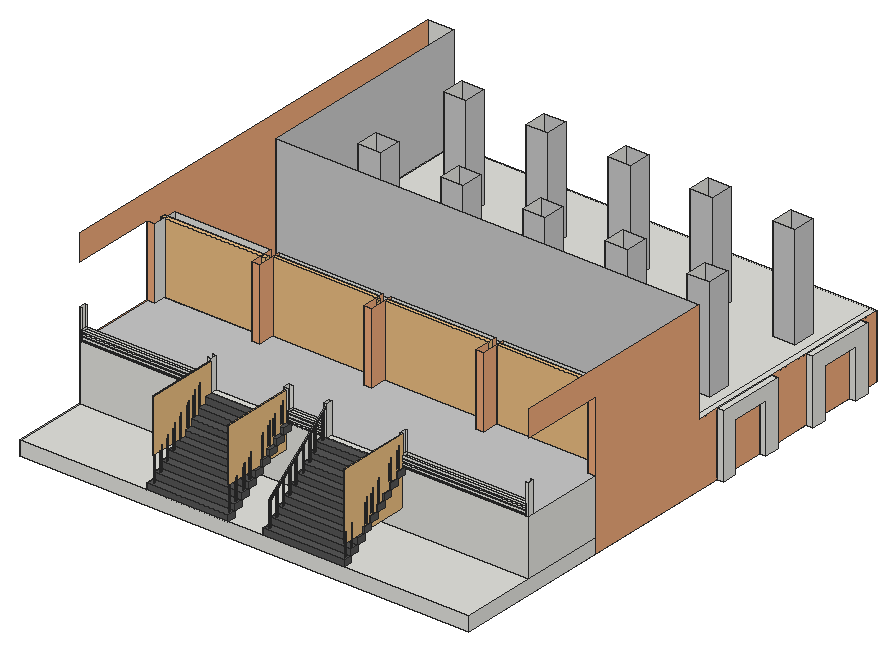
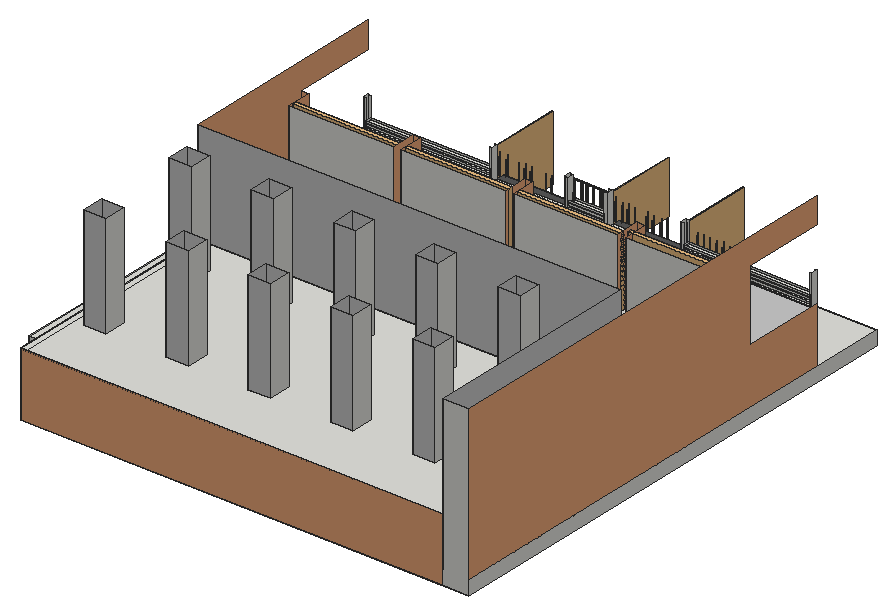
# SketchUp Ruby script. Lengths in inches.
U = 1.inch
M = Sketchup.active_model
def pt(a) = Geom::Point3d.new(a.map { |v| v * U })
def face(e, loops, mat)
  f = e.add_face(loops[0].map { |a| pt(a) })
  loops[1..].each { |l| e.add_face(l.map { |a| pt(a) }).erase! }
  f.material = f.back_material = mat if mat
  f
end
# faces: each face lists its corners as indices into pts; further lists are holes
def faces(e, pts, list, mat = nil) = list.each { |f| face(e, (f[0].is_a?(Array) ? f : [f]).map { |l| l.map { |i| pts[i] } }, mat) }
# xy, xz, yz: faces in a plane at the given z, y or x. An outline is a flat list of corners, or four numbers for a rectangle; further outlines are holes
def ring(l) = l.size == 4 ? [[l[0], l[1]], [l[2], l[1]], [l[2], l[3]], [l[0], l[3]]] : l.each_slice(2).to_a
def flat(e, list, mat, &to3) = list.each { |f| face(e, (f[0].is_a?(Array) ? f : [f]).map { |l| ring(l).map { |u, v| to3.(u, v) } }, mat) }
def xy(e, z, list, mat = nil) = flat(e, list, mat) { |x, y| [x, y, z] }
def xz(e, y, list, mat = nil) = flat(e, list, mat) { |x, z| [x, y, z] }
def yz(e, x, list, mat = nil) = flat(e, list, mat) { |y, z| [x, y, z] }
def lines(e, pts, list) = list.each { |a, b| e.add_line(pt(pts[a]), pt(pts[b])) }
# prism: a flat outline (further loops are holes) pulled along v
def prism(e, loops, v, mat = nil)
  f = face(e, loops, mat); d = Geom::Vector3d.new(v.map { |x| x * U })
  f.pushpull(f.normal.samedirection?(d) ? d.length : -d.length)
end
def box(e, o, s, mat = nil) = prism(e, [[o, [o[0] + s[0], o[1], o[2]], [o[0] + s[0], o[1] + s[1], o[2]], [o[0], o[1] + s[1], o[2]]]], [0, 0, s[2]], mat)
def at(x, y, z, deg = 0) = Geom::Transformation.translation(pt([x, y, z])) * Geom::Transformation.rotation(ORIGIN, Z_AXIS, deg.degrees)
def axes(o, x, y, z) = Geom::Transformation.new([*x, 0, *y, 0, *z, 0, *pt(o).to_a, 1])
def part(name) = M.definitions.add(name)
# library, detail: a bought-in or finely detailed component or shape, given as its bounding box
def library(name, o, s) = part(name).tap { |d| box(d.entities, o, s) }
def detail(e, o, s) = box(e.add_group.entities, o, s)
def put(e, d, t, mat = nil) = e.add_instance(d, t).tap { |i| i.material = mat if mat }
def group(e, t, mat = nil) = e.add_group.tap { |g| g.transformation = t; g.material = mat if mat }.entities
root = M.entities
M.materials.add("Generic\#1").color = [236, 168, 122]
M.materials.add("Generic\#4").color = [201, 201, 201]
M.materials.add("[Color M06]").color = [86, 86, 86]
c1 = part("Group\#6")
xy(c1.entities,0,[[0,0,123.875,12.625]])
xy(c1.entities,9.4375,[[0,0,123.875,12.625]])
xz(c1.entities,0,[[0,0,123.875,9.4375]])
yz(c1.entities,0,[[0,0,12.625,9.4375]])
yz(c1.entities,123.875,[[0,0,12.625,9.4375]])
c2 = library("Group\#7",[0,0,0],[158.4375,6,107.5625])
prism(root,[[[214.39,5.8,-54.75],[214.29,6.05,-54.75],[214.26,6.3,-54.75],[214.29,6.5625,-54.75],[214.39,6.8,-54.75],[214.55,7.01,-54.75],[214.76,7.17,-54.75],[215,7.27,-54.75],[215.26,7.3,-54.75],[215.52,7.27,-54.75],[215.76,7.17,-54.75],[215.97,7.01,-54.75],[216.125,6.8,-54.75],[216.23,6.5625,-54.75],[216.26,6.3,-54.75],[216.23,6.05,-54.75],[216.125,5.8,-54.75],[215.97,5.6,-54.75],[215.76,5.4375,-54.75],[215.52,5.34,-54.75],[215.26,5.3,-54.75],[215,5.34,-54.75],[214.76,5.4375,-54.75],[214.55,5.6,-54.75]]],[0,0,37.69])
prism(root,[[[329.63,5.9375,-54.75],[329.39,5.84,-54.75],[329.13,5.8,-54.75],[328.875,5.84,-54.75],[328.63,5.9375,-54.75],[328.43,6.1,-54.75],[328.27,6.3,-54.75],[328.17,6.55,-54.75],[328.13,6.8,-54.75],[328.17,7.0625,-54.75],[328.27,7.3,-54.75],[328.43,7.51,-54.75],[328.63,7.67,-54.75],[328.875,7.77,-54.75],[329.13,7.8,-54.75],[329.39,7.77,-54.75],[329.63,7.67,-54.75],[329.84,7.51,-54.75],[330,7.3,-54.75],[330.1,7.0625,-54.75],[330.13,6.8,-54.75],[330.1,6.55,-54.75],[330,6.3,-54.75],[329.84,6.1,-54.75]]],[0,0,38.25])
prism(root,[[[390.83,7.14,-54.75],[391.07,7.25,-54.75],[391.32,7.3,-54.75],[391.58,7.28,-54.75],[391.83,7.2,-54.75],[392.05,7.05,-54.75],[392.22,6.86,-54.75],[392.33,6.625,-54.75],[392.38,6.37,-54.75],[392.36,6.11,-54.75],[392.28,5.86,-54.75],[392.13,5.64,-54.75],[391.9375,5.47,-54.75],[391.7,5.36,-54.75],[391.45,5.31,-54.75],[391.1875,5.32,-54.75],[390.94,5.41,-54.75],[390.72,5.55,-54.75],[390.55,5.75,-54.75],[390.4375,5.98,-54.75],[390.39,6.24,-54.75],[390.4,6.5,-54.75],[390.49,6.75,-54.75],[390.63,6.97,-54.75]]],[0,0,38.17])
prism(root,[[[505.97,6.1,-54.75],[505.76,5.9375,-54.75],[505.52,5.84,-54.75],[505.26,5.8,-54.75],[505,5.84,-54.75],[504.76,5.9375,-54.75],[504.55,6.1,-54.75],[504.39,6.3,-54.75],[504.29,6.55,-54.75],[504.26,6.8,-54.75],[504.29,7.0625,-54.75],[504.39,7.3,-54.75],[504.55,7.51,-54.75],[504.76,7.67,-54.75],[505,7.77,-54.75],[505.26,7.8,-54.75],[505.52,7.77,-54.75],[505.76,7.67,-54.75],[505.97,7.51,-54.75],[506.125,7.3,-54.75],[506.23,7.0625,-54.75],[506.26,6.8,-54.75],[506.23,6.55,-54.75],[506.125,6.3,-54.75]]],[0,0,38.28])
prism(root,[[[214.55,18.28,-45.3125],[214.39,18.49,-45.3125],[214.29,18.73,-45.3125],[214.26,18.99,-45.3125],[214.29,19.25,-45.3125],[214.39,19.49,-45.3125],[214.55,19.7,-45.3125],[214.76,19.86,-45.3125],[215,19.96,-45.3125],[215.26,19.99,-45.3125],[215.52,19.96,-45.3125],[215.76,19.86,-45.3125],[215.97,19.7,-45.3125],[216.125,19.49,-45.3125],[216.22,19.25,-45.3125],[216.26,18.99,-45.3125],[216.22,18.73,-45.3125],[216.125,18.49,-45.3125],[215.97,18.28,-45.3125],[215.76,18.125,-45.3125],[215.52,18.03,-45.3125],[215.26,17.99,-45.3125],[215,18.03,-45.3125],[214.76,18.125,-45.3125]]],[0,0,36.6875])
prism(root,[[[329.39,17.59,-45.3125],[329.13,17.55,-45.3125],[328.875,17.59,-45.3125],[328.63,17.6875,-45.3125],[328.43,17.85,-45.3125],[328.27,18.05,-45.3125],[328.17,18.3,-45.3125],[328.13,18.55,-45.3125],[328.17,18.8125,-45.3125],[328.27,19.05,-45.3125],[328.43,19.26,-45.3125],[328.63,19.42,-45.3125],[328.875,19.52,-45.3125],[329.13,19.55,-45.3125],[329.39,19.52,-45.3125],[329.63,19.42,-45.3125],[329.84,19.26,-45.3125],[330,19.05,-45.3125],[330.1,18.8125,-45.3125],[330.13,18.55,-45.3125],[330.1,18.3,-45.3125],[330,18.05,-45.3125],[329.84,17.85,-45.3125],[329.63,17.6875,-45.3125]]],[0,0,36.6875])
prism(root,[[[390.68,19.7,-45.3125],[390.88,19.86,-45.3125],[391.125,19.96,-45.3125],[391.38,19.99,-45.3125],[391.64,19.96,-45.3125],[391.88,19.86,-45.3125],[392.09,19.7,-45.3125],[392.25,19.49,-45.3125],[392.35,19.25,-45.3125],[392.38,18.99,-45.3125],[392.35,18.73,-45.3125],[392.25,18.49,-45.3125],[392.09,18.28,-45.3125],[391.88,18.125,-45.3125],[391.64,18.03,-45.3125],[391.38,17.99,-45.3125],[391.125,18.03,-45.3125],[390.88,18.125,-45.3125],[390.68,18.28,-45.3125],[390.52,18.49,-45.3125],[390.42,18.73,-45.3125],[390.38,18.99,-45.3125],[390.42,19.25,-45.3125],[390.52,19.49,-45.3125]]],[0,0,37.04])
prism(root,[[[505.26,17.55,-45.3125],[505,17.59,-45.3125],[504.76,17.6875,-45.3125],[504.55,17.85,-45.3125],[504.39,18.05,-45.3125],[504.29,18.3,-45.3125],[504.26,18.55,-45.3125],[504.29,18.8125,-45.3125],[504.39,19.05,-45.3125],[504.55,19.26,-45.3125],[504.76,19.42,-45.3125],[505,19.52,-45.3125],[505.26,19.55,-45.3125],[505.52,19.52,-45.3125],[505.76,19.42,-45.3125],[505.97,19.26,-45.3125],[506.125,19.05,-45.3125],[506.22,18.8125,-45.3125],[506.26,18.55,-45.3125],[506.22,18.3,-45.3125],[506.125,18.05,-45.3125],[505.97,17.85,-45.3125],[505.76,17.6875,-45.3125],[505.52,17.59,-45.3125]]],[0,0,36.61])
prism(root,[[[216.26,31.24,-35.875],[216.22,30.98,-35.875],[216.125,30.74,-35.875],[215.96,30.53,-35.875],[215.76,30.375,-35.875],[215.52,30.28,-35.875],[215.26,30.24,-35.875],[215,30.28,-35.875],[214.76,30.375,-35.875],[214.55,30.53,-35.875],[214.39,30.74,-35.875],[214.29,30.98,-35.875],[214.26,31.24,-35.875],[214.29,31.5,-35.875],[214.39,31.74,-35.875],[214.55,31.95,-35.875],[214.76,32.11,-35.875],[215,32.21,-35.875],[215.26,32.24,-35.875],[215.52,32.21,-35.875],[215.76,32.11,-35.875],[215.96,31.95,-35.875],[216.125,31.74,-35.875],[216.22,31.5,-35.875]]],[0,0,36.6875])
prism(root,[[[329.39,34.64,-35.875],[329.63,34.54,-35.875],[329.84,34.39,-35.875],[330,34.18,-35.875],[330.1,33.9375,-35.875],[330.13,33.68,-35.875],[330.1,33.42,-35.875],[330,33.18,-35.875],[329.84,32.97,-35.875],[329.63,32.8125,-35.875],[329.39,32.71,-35.875],[329.13,32.68,-35.875],[328.875,32.71,-35.875],[328.63,32.8125,-35.875],[328.43,32.97,-35.875],[328.27,33.18,-35.875],[328.17,33.42,-35.875],[328.13,33.68,-35.875],[328.17,33.9375,-35.875],[328.27,34.18,-35.875],[328.43,34.39,-35.875],[328.63,34.54,-35.875],[328.875,34.64,-35.875],[329.13,34.68,-35.875]]],[0,0,38.36])
prism(root,[[[392.11,31.93,-35.875],[392.26,31.72,-35.875],[392.35,31.47,-35.875],[392.38,31.22,-35.875],[392.34,30.96,-35.875],[392.24,30.72,-35.875],[392.07,30.52,-35.875],[391.86,30.36,-35.875],[391.62,30.27,-35.875],[391.36,30.24,-35.875],[391.1,30.28,-35.875],[390.86,30.39,-35.875],[390.66,30.55,-35.875],[390.5,30.76,-35.875],[390.41,31.01,-35.875],[390.38,31.27,-35.875],[390.42,31.52,-35.875],[390.53,31.76,-35.875],[390.69,31.97,-35.875],[390.91,32.12,-35.875],[391.15,32.21,-35.875],[391.41,32.24,-35.875],[391.67,32.2,-35.875],[391.9,32.09,-35.875]]],[0,0,36.39])
prism(root,[[[215,43.02,-26.4375],[214.76,43.125,-26.4375],[214.55,43.28,-26.4375],[214.39,43.49,-26.4375],[214.29,43.73,-26.4375],[214.26,43.99,-26.4375],[214.29,44.25,-26.4375],[214.39,44.49,-26.4375],[214.55,44.7,-26.4375],[214.76,44.86,-26.4375],[215,44.96,-26.4375],[215.26,44.99,-26.4375],[215.52,44.96,-26.4375],[215.76,44.86,-26.4375],[215.96,44.7,-26.4375],[216.12,44.49,-26.4375],[216.22,44.25,-26.4375],[216.26,43.99,-26.4375],[216.22,43.73,-26.4375],[216.12,43.49,-26.4375],[215.96,43.28,-26.4375],[215.76,43.125,-26.4375],[215.52,43.02,-26.4375],[215.26,42.99,-26.4375]]],[0,0,36.6875])
prism(root,[[[328.13,45.68,-26.4375],[328.17,45.9375,-26.4375],[328.27,46.18,-26.4375],[328.42,46.39,-26.4375],[328.63,46.54,-26.4375],[328.87,46.64,-26.4375],[329.13,46.68,-26.4375],[329.39,46.64,-26.4375],[329.63,46.54,-26.4375],[329.84,46.39,-26.4375],[330,46.18,-26.4375],[330.1,45.9375,-26.4375],[330.13,45.68,-26.4375],[330.1,45.42,-26.4375],[330,45.18,-26.4375],[329.84,44.97,-26.4375],[329.63,44.8125,-26.4375],[329.39,44.71,-26.4375],[329.13,44.68,-26.4375],[328.87,44.71,-26.4375],[328.63,44.8125,-26.4375],[328.42,44.97,-26.4375],[328.27,45.18,-26.4375],[328.17,45.42,-26.4375]]],[0,0,38.36])
prism(root,[[[391.38,42.99,-26.4375],[391.12,43.02,-26.4375],[390.88,43.125,-26.4375],[390.67,43.28,-26.4375],[390.52,43.49,-26.4375],[390.42,43.73,-26.4375],[390.38,43.99,-26.4375],[390.42,44.25,-26.4375],[390.52,44.49,-26.4375],[390.67,44.7,-26.4375],[390.88,44.86,-26.4375],[391.12,44.96,-26.4375],[391.38,44.99,-26.4375],[391.64,44.96,-26.4375],[391.88,44.86,-26.4375],[392.09,44.7,-26.4375],[392.25,44.49,-26.4375],[392.35,44.25,-26.4375],[392.38,43.99,-26.4375],[392.35,43.73,-26.4375],[392.25,43.49,-26.4375],[392.09,43.28,-26.4375],[391.88,43.125,-26.4375],[391.64,43.02,-26.4375]]],[0,0,37.3125])
prism(root,[[[506.22,45.9375,-26.4375],[506.26,45.68,-26.4375],[506.22,45.42,-26.4375],[506.12,45.18,-26.4375],[505.96,44.97,-26.4375],[505.76,44.8125,-26.4375],[505.52,44.71,-26.4375],[505.26,44.68,-26.4375],[505,44.71,-26.4375],[504.76,44.8125,-26.4375],[504.55,44.97,-26.4375],[504.39,45.18,-26.4375],[504.29,45.42,-26.4375],[504.26,45.68,-26.4375],[504.29,45.9375,-26.4375],[504.39,46.18,-26.4375],[504.55,46.39,-26.4375],[504.76,46.54,-26.4375],[505,46.64,-26.4375],[505.26,46.68,-26.4375],[505.52,46.64,-26.4375],[505.76,46.54,-26.4375],[505.96,46.39,-26.4375],[506.12,46.18,-26.4375]]],[0,0,37.92])
prism(root,[[[391.77,6.06,-17.3],[391.96,6,-17.22],[392.11,5.93,-17.13],[392.19,5.85,-17.02],[392.22,5.76,-16.9],[392.18,5.68,-16.78],[392.08,5.6,-16.67],[391.92,5.53,-16.58],[391.72,5.47,-16.51],[391.49,5.44,-16.47],[391.24,5.43,-16.46],[391,5.44,-16.48],[390.77,5.48,-16.52],[390.58,5.53,-16.6],[390.43,5.6,-16.7],[390.34,5.6875,-16.81],[390.32,5.77,-16.92],[390.35,5.86,-17.04],[390.46,5.94,-17.15],[390.61,6.01,-17.24],[390.8125,6.0625,-17.3125],[391.05,6.09,-17.35],[391.29,6.1,-17.37],[391.54,6.09,-17.35]]],[-0.53,106.82,78.87])
prism(root,[[[215.96,55.03,-17],[215.76,54.875,-17],[215.51,54.77,-17],[215.26,54.74,-17],[215,54.77,-17],[214.76,54.875,-17],[214.55,55.03,-17],[214.39,55.24,-17],[214.29,55.48,-17],[214.26,55.74,-17],[214.29,56,-17],[214.39,56.24,-17],[214.55,56.45,-17],[214.76,56.61,-17],[215,56.71,-17],[215.26,56.74,-17],[215.51,56.71,-17],[215.76,56.61,-17],[215.96,56.45,-17],[216.12,56.24,-17],[216.22,56,-17],[216.26,55.74,-17],[216.22,55.48,-17],[216.12,55.24,-17]]],[0,0,36.25])
prism(root,[[[504.76,56.8125,-17],[504.55,56.97,-17],[504.39,57.18,-17],[504.29,57.42,-17],[504.26,57.68,-17],[504.29,57.9375,-17],[504.39,58.18,-17],[504.55,58.39,-17],[504.76,58.54,-17],[505,58.64,-17],[505.26,58.68,-17],[505.51,58.64,-17],[505.76,58.54,-17],[505.96,58.39,-17],[506.12,58.18,-17],[506.22,57.9375,-17],[506.26,57.68,-17],[506.22,57.42,-17],[506.12,57.18,-17],[505.96,56.97,-17],[505.76,56.8125,-17],[505.51,56.71,-17],[505.26,56.68,-17],[505,56.71,-17]]],[0,0,37.02])
prism(root,[[[392.25,55.24,-17],[392.09,55.03,-17],[391.88,54.875,-17],[391.64,54.77,-17],[391.38,54.74,-17],[391.12,54.77,-17],[390.88,54.875,-17],[390.67,55.03,-17],[390.51,55.24,-17],[390.41,55.48,-17],[390.38,55.74,-17],[390.41,56,-17],[390.51,56.24,-17],[390.67,56.45,-17],[390.88,56.61,-17],[391.12,56.71,-17],[391.38,56.74,-17],[391.64,56.71,-17],[391.88,56.61,-17],[392.09,56.45,-17],[392.25,56.24,-17],[392.35,56,-17],[392.38,55.74,-17],[392.35,55.48,-17]]],[0,0,35.9375])
prism(root,[[[215,68.71,-7.5625],[214.75,68.8125,-7.5625],[214.55,68.97,-7.5625],[214.39,69.18,-7.5625],[214.29,69.42,-7.5625],[214.25,69.68,-7.5625],[214.29,69.9375,-7.5625],[214.39,70.18,-7.5625],[214.55,70.38,-7.5625],[214.75,70.54,-7.5625],[215,70.64,-7.5625],[215.25,70.68,-7.5625],[215.51,70.64,-7.5625],[215.75,70.54,-7.5625],[215.96,70.38,-7.5625],[216.12,70.18,-7.5625],[216.22,69.9375,-7.5625],[216.25,69.68,-7.5625],[216.22,69.42,-7.5625],[216.12,69.18,-7.5625],[215.96,68.97,-7.5625],[215.75,68.8125,-7.5625],[215.51,68.71,-7.5625],[215.25,68.68,-7.5625]]],[0,0,36.43])
prism(root,[[[330.11,69.68,-7.5625],[330.07,69.42,-7.5625],[329.98,69.1875,-7.5625],[329.82,68.99,-7.5625],[329.62,68.83,-7.5625],[329.38,68.73,-7.5625],[329.13,68.7,-7.5625],[328.875,68.73,-7.5625],[328.64,68.83,-7.5625],[328.4375,68.99,-7.5625],[328.28,69.1875,-7.5625],[328.1875,69.42,-7.5625],[328.15,69.68,-7.5625],[328.1875,69.93,-7.5625],[328.28,70.17,-7.5625],[328.4375,70.37,-7.5625],[328.64,70.52,-7.5625],[328.875,70.62,-7.5625],[329.13,70.65,-7.5625],[329.38,70.62,-7.5625],[329.62,70.52,-7.5625],[329.82,70.37,-7.5625],[329.98,70.17,-7.5625],[330.07,69.93,-7.5625]]],[0,0,36.6875])
prism(root,[[[392.09,68.97,-7.5625],[391.88,68.8125,-7.5625],[391.64,68.71,-7.5625],[391.38,68.68,-7.5625],[391.12,68.71,-7.5625],[390.88,68.8125,-7.5625],[390.67,68.97,-7.5625],[390.51,69.18,-7.5625],[390.41,69.42,-7.5625],[390.38,69.68,-7.5625],[390.41,69.9375,-7.5625],[390.51,70.18,-7.5625],[390.67,70.38,-7.5625],[390.88,70.54,-7.5625],[391.12,70.64,-7.5625],[391.38,70.68,-7.5625],[391.64,70.64,-7.5625],[391.88,70.54,-7.5625],[392.09,70.38,-7.5625],[392.25,70.18,-7.5625],[392.35,69.9375,-7.5625],[392.38,69.68,-7.5625],[392.35,69.42,-7.5625],[392.25,69.18,-7.5625]]],[0,0,36.4])
prism(root,[[[505,68.71,-7.5625],[504.75,68.8125,-7.5625],[504.55,68.97,-7.5625],[504.39,69.18,-7.5625],[504.29,69.42,-7.5625],[504.25,69.68,-7.5625],[504.29,69.9375,-7.5625],[504.39,70.18,-7.5625],[504.55,70.38,-7.5625],[504.75,70.54,-7.5625],[505,70.64,-7.5625],[505.25,70.68,-7.5625],[505.51,70.64,-7.5625],[505.75,70.54,-7.5625],[505.96,70.38,-7.5625],[506.12,70.18,-7.5625],[506.22,69.9375,-7.5625],[506.25,69.68,-7.5625],[506.22,69.42,-7.5625],[506.12,69.18,-7.5625],[505.96,68.97,-7.5625],[505.75,68.8125,-7.5625],[505.51,68.71,-7.5625],[505.25,68.68,-7.5625]]],[0,0,36.75])
prism(root,[[[216.22,81.42,1.875],[216.12,81.18,1.875],[215.96,80.97,1.875],[215.75,80.8125,1.875],[215.51,80.71,1.875],[215.25,80.68,1.875],[215,80.71,1.875],[214.75,80.8125,1.875],[214.55,80.97,1.875],[214.39,81.18,1.875],[214.29,81.42,1.875],[214.25,81.68,1.875],[214.29,81.9375,1.875],[214.39,82.18,1.875],[214.55,82.38,1.875],[214.75,82.54,1.875],[215,82.64,1.875],[215.25,82.68,1.875],[215.51,82.64,1.875],[215.75,82.54,1.875],[215.96,82.38,1.875],[216.12,82.18,1.875],[216.22,81.9375,1.875],[216.25,81.68,1.875]]],[0,0,36.25])
prism(root,[[[328.87,82.64,1.875],[329.13,82.68,1.875],[329.39,82.64,1.875],[329.63,82.54,1.875],[329.84,82.38,1.875],[329.99,82.18,1.875],[330.09,81.9375,1.875],[330.13,81.68,1.875],[330.09,81.42,1.875],[329.99,81.18,1.875],[329.84,80.97,1.875],[329.63,80.8125,1.875],[329.39,80.71,1.875],[329.13,80.68,1.875],[328.87,80.71,1.875],[328.63,80.8125,1.875],[328.42,80.97,1.875],[328.26,81.18,1.875],[328.16,81.42,1.875],[328.13,81.68,1.875],[328.16,81.9375,1.875],[328.26,82.18,1.875],[328.42,82.38,1.875],[328.63,82.54,1.875]]],[0,0,36.6875])
prism(root,[[[390.88,80.8125,1.875],[390.67,80.97,1.875],[390.51,81.18,1.875],[390.41,81.42,1.875],[390.38,81.68,1.875],[390.41,81.9375,1.875],[390.51,82.18,1.875],[390.67,82.38,1.875],[390.88,82.54,1.875],[391.12,82.64,1.875],[391.38,82.68,1.875],[391.64,82.64,1.875],[391.88,82.54,1.875],[392.09,82.38,1.875],[392.24,82.18,1.875],[392.34,81.9375,1.875],[392.38,81.68,1.875],[392.34,81.42,1.875],[392.24,81.18,1.875],[392.09,80.97,1.875],[391.88,80.8125,1.875],[391.64,80.71,1.875],[391.38,80.68,1.875],[391.12,80.71,1.875]]],[0,0,36.25])
prism(root,[[[215.91,92,11.3125],[215.8125,91.76,11.3125],[215.66,91.55,11.3125],[215.45,91.39,11.3125],[215.21,91.29,11.3125],[214.95,91.26,11.3125],[214.69,91.29,11.3125],[214.45,91.39,11.3125],[214.24,91.55,11.3125],[214.08,91.76,11.3125],[213.98,92,11.3125],[213.95,92.26,11.3125],[213.98,92.52,11.3125],[214.08,92.76,11.3125],[214.24,92.96,11.3125],[214.45,93.12,11.3125],[214.69,93.22,11.3125],[214.95,93.26,11.3125],[215.21,93.22,11.3125],[215.45,93.12,11.3125],[215.66,92.96,11.3125],[215.8125,92.76,11.3125],[215.91,92.52,11.3125],[215.95,92.26,11.3125]]],[0,0,34.8125])
prism(root,[[[328.32,93.12,11.3125],[328.56,93.22,11.3125],[328.82,93.26,11.3125],[329.08,93.22,11.3125],[329.32,93.12,11.3125],[329.53,92.96,11.3125],[329.6875,92.76,11.3125],[329.79,92.52,11.3125],[329.82,92.26,11.3125],[329.79,92,11.3125],[329.6875,91.76,11.3125],[329.53,91.55,11.3125],[329.32,91.39,11.3125],[329.08,91.29,11.3125],[328.82,91.26,11.3125],[328.56,91.29,11.3125],[328.32,91.39,11.3125],[328.12,91.55,11.3125],[327.96,91.76,11.3125],[327.86,92,11.3125],[327.82,92.26,11.3125],[327.86,92.52,11.3125],[327.96,92.76,11.3125],[328.12,92.96,11.3125]]],[0,0,34.875])
prism(root,[[[392.04,92.52,11.3125],[392.07,92.26,11.3125],[392.04,92,11.3125],[391.9375,91.76,11.3125],[391.78,91.55,11.3125],[391.57,91.39,11.3125],[391.33,91.29,11.3125],[391.07,91.26,11.3125],[390.81,91.29,11.3125],[390.57,91.39,11.3125],[390.37,91.55,11.3125],[390.21,91.76,11.3125],[390.11,92,11.3125],[390.07,92.26,11.3125],[390.11,92.52,11.3125],[390.21,92.76,11.3125],[390.37,92.96,11.3125],[390.57,93.12,11.3125],[390.81,93.22,11.3125],[391.07,93.26,11.3125],[391.33,93.22,11.3125],[391.57,93.12,11.3125],[391.78,92.96,11.3125],[391.9375,92.76,11.3125]]],[0,0,34.93])
prism(root,[[[504.08,91.76,11.3125],[503.98,92,11.3125],[503.95,92.26,11.3125],[503.98,92.52,11.3125],[504.08,92.76,11.3125],[504.24,92.96,11.3125],[504.45,93.12,11.3125],[504.69,93.22,11.3125],[504.95,93.26,11.3125],[505.21,93.22,11.3125],[505.45,93.12,11.3125],[505.66,92.96,11.3125],[505.8125,92.76,11.3125],[505.91,92.52,11.3125],[505.95,92.26,11.3125],[505.91,92,11.3125],[505.8125,91.76,11.3125],[505.66,91.55,11.3125],[505.45,91.39,11.3125],[505.21,91.29,11.3125],[504.95,91.26,11.3125],[504.69,91.29,11.3125],[504.45,91.39,11.3125],[504.24,91.55,11.3125]]],[0,0,34.98])
prism(root,[[[329.0625,106.45,20.75],[328.82,106.35,20.75],[328.5625,106.3125,20.75],[328.3,106.35,20.75],[328.0625,106.45,20.75],[327.86,106.61,20.75],[327.7,106.8125,20.75],[327.6,107.05,20.75],[327.5625,107.3125,20.75],[327.6,107.57,20.75],[327.7,107.8125,20.75],[327.86,108.02,20.75],[328.0625,108.18,20.75],[328.3,108.28,20.75],[328.5625,108.3125,20.75],[328.82,108.28,20.75],[329.0625,108.18,20.75],[329.27,108.02,20.75],[329.43,107.8125,20.75],[329.53,107.57,20.75],[329.5625,107.3125,20.75],[329.53,107.05,20.75],[329.43,106.8125,20.75],[329.27,106.61,20.75]]],[0,0,36.6875])
prism(root,[[[390.55,106.33,20.75],[390.3,106.43,20.75],[390.09,106.59,20.75],[389.93,106.8,20.75],[389.83,107.05,20.75],[389.8,107.3125,20.75],[389.83,107.58,20.75],[389.93,107.82,20.75],[390.09,108.03,20.75],[390.3,108.19,20.75],[390.55,108.29,20.75],[390.8125,108.33,20.75],[391.08,108.29,20.75],[391.32,108.19,20.75],[391.53,108.03,20.75],[391.69,107.82,20.75],[391.79,107.58,20.75],[391.83,107.3125,20.75],[391.79,107.05,20.75],[391.69,106.8,20.75],[391.53,106.59,20.75],[391.32,106.43,20.75],[391.08,106.33,20.75],[390.8125,106.3,20.75]]],[0,0,36.25])
prism(root,[[[505.6875,107.3125,20.75],[505.65,107.05,20.75],[505.55,106.8125,20.75],[505.39,106.61,20.75],[505.1875,106.45,20.75],[504.95,106.35,20.75],[504.6875,106.3125,20.75],[504.43,106.35,20.75],[504.1875,106.45,20.75],[503.98,106.61,20.75],[503.82,106.8125,20.75],[503.72,107.05,20.75],[503.6875,107.3125,20.75],[503.72,107.57,20.75],[503.82,107.8125,20.75],[503.98,108.02,20.75],[504.1875,108.18,20.75],[504.43,108.28,20.75],[504.6875,108.3125,20.75],[504.95,108.28,20.75],[505.1875,108.18,20.75],[505.39,108.02,20.75],[505.55,107.8125,20.75],[505.65,107.57,20.75]]],[0,0,36.25])
xy(root,-85.875,[[16.6875,0,698.4375,774.8125],[698.4375,471.86,708.4375,494.03],[698.4375,553.18,708.4375,575.34],[698.4375,641.74,708.4375,663.9],[698.4375,723.05,708.4375,745.22]])
xy(root,-64.1875,[[16.6875,0,698.4375,113.625]])
xy(root,-11.125,[[698.4375,494.03,708.4375,553.18],[698.4375,663.9,708.4375,723.05]])
xy(root,11.5625,[[[56.125,437.0625,689.4375,774.8125],[640.76,649.6,674.95,683.79],[515.63,649.6,549.82,683.79],[390.51,649.6,424.7,683.79],[265.38,649.6,299.57,683.79],[140.26,649.6,174.45,683.79],[640.76,487.6,674.95,521.79],[515.63,487.6,549.82,521.79],[390.51,487.6,424.7,521.79],[265.38,487.6,299.57,521.79],[140.26,487.6,174.45,521.79]],[689.4375,437.0625,698.4375,774.8125],[698.4375,471.86,708.4375,575.34],[140.26,487.6,174.45,521.79],[265.38,487.6,299.57,521.79],
  [390.51,487.6,424.7,521.79],[515.63,487.6,549.82,521.79],[640.76,487.6,674.95,521.79],[698.4375,641.74,708.4375,745.22],[140.26,649.6,174.45,683.79],
  [265.38,649.6,299.57,683.79],[390.51,649.6,424.7,683.79],[515.63,649.6,549.82,683.79],[640.76,649.6,674.95,683.79]])
xy(root,20.75,[[16.6875,113.625,19.375,122.8125],[19.375,113.625,211.0625,122.8125],[211.0625,113.625,215.625,122.8125],[215.625,113.625,327,122.8125],[327,113.625,332.7,122.8125],
  [332.7,113.625,387.61,122.8125],[387.61,113.625,391.97,122.8125],[391.97,113.625,502.82,122.8125],[502.82,113.625,505.65,122.8125],[505.65,113.625,694.3125,122.8125],
  [694.3125,113.625,698.4375,122.8125]])
xy(root,20.75,[[16.6875,122.8125,698.4375,122.8125,698.4375,241.3125,686.4375,241.3125,686.4375,278.75,528,278.75,528,241.3125,516,241.3125,516,278.75,357.5625,278.75,357.5625,241.3125,345.5625,241.3125,345.5625,278.75,187.125,278.75,187.125,241.3125,175.125,241.3125,175.125,278.75,28.6875,278.75,28.6875,241.3125,16.6875,241.3125]],"Generic\#4")
xy(root,22.0625,[[19.375,113.625,211.0625,122.8125],[332.7,113.625,387.61,122.8125],[505.65,113.625,694.3125,122.8125]])
xy(root,24.0625,[[19.375,113.625,211.0625,122.8125],[332.7,113.625,387.73,122.8125],[505.65,113.625,694.3125,122.8125]])
xy(root,27.0625,[[19.375,113.625,211.0625,122.8125],[332.7,113.625,387.73,122.8125],[505.65,113.625,694.3125,122.8125]])
xy(root,29.0625,[[19.375,113.625,211.0625,122.8125],[332.7,113.625,387.73,122.8125],[505.65,113.625,694.3125,122.8125]])
xy(root,32.0625,[[19.375,113.625,211.0625,122.8125],[332.7,113.625,387.73,122.8125],[505.65,113.625,694.3125,122.8125]])
xy(root,34.0625,[[19.375,113.625,211.0625,122.8125],[332.7,113.625,387.73,122.8125],[505.65,113.625,694.3125,122.8125]])
xz(root,0,[[16.6875,-85.875,698.4375,-64.1875]])
xz(root,113.625,[[16.6875,-64.1875,698.4375,-64.1875,698.4375,20.75,336.6875,20.75,336.6875,11.3125,212.8125,11.3125,212.8125,20.75,16.6875,20.75],[212.8125,11.3125,336.6875,20.75],[16.6875,20.75,19.375,67.0625],[19.375,20.75,211.0625,22.0625],[211.0625,20.75,215.625,67.0625],
  [327,20.75,332.7,67.0625],[332.7,20.75,387.61,22.0625],[387.61,20.75,391.97,20.75,391.97,67.0625,387.61,67.0625,387.61,62.0625,387.73,62.0625,387.73,59.0625,387.61,59.0625,387.61,57.0625,387.73,57.0625,387.73,54.0625,387.61,54.0625,387.61,52.0625,387.73,52.0625,387.73,49.0625,387.61,49.0625,387.61,47.0625,387.73,47.0625,387.73,44.0625,387.61,44.0625,387.61,42.0625,387.73,42.0625,387.73,39.0625,387.61,39.0625,387.61,37.0625,387.73,37.0625,387.73,34.0625,387.61,34.0625,387.61,32.0625,387.73,32.0625,387.73,29.0625,387.61,29.0625,387.61,27.0625,387.73,27.0625,387.73,24.0625,387.61,24.0625],[502.82,20.75,505.65,20.75,505.65,64.0625,505.5625,64.0625,505.5625,67.0625,502.82,67.0625],[505.65,20.75,694.3125,22.0625],
  [694.3125,20.75,698.4375,67.0625],[19.375,24.0625,211.0625,27.0625],[332.7,24.0625,387.61,27.0625],[387.61,24.0625,387.73,27.0625],[505.65,24.0625,694.3125,27.0625],
  [19.375,29.0625,211.0625,32.0625],[332.7,29.0625,387.61,32.0625],[387.61,29.0625,387.73,32.0625],[505.65,29.0625,694.3125,32.0625],[19.375,34.0625,211.0625,37.0625],
  [332.7,34.0625,387.61,37.0625],[387.61,34.0625,387.73,37.0625],[505.65,34.0625,694.3125,37.0625]])
xz(root,122.8125,[[16.6875,20.75,19.375,67.0625],[19.375,20.75,211.0625,22.0625],[211.0625,20.75,215.625,67.0625],[327,20.75,332.7,67.0625],[332.7,20.75,387.61,22.0625],
  [387.61,20.75,387.61,24.0625,387.73,24.0625,387.73,27.0625,387.61,27.0625,387.61,29.0625,387.73,29.0625,387.73,32.0625,387.61,32.0625,387.61,34.0625,387.73,34.0625,387.73,37.0625,387.61,37.0625,387.61,39.0625,387.73,39.0625,387.73,42.0625,387.61,42.0625,387.61,44.0625,387.73,44.0625,387.73,47.0625,387.61,47.0625,387.61,49.0625,387.73,49.0625,387.73,52.0625,387.61,52.0625,387.61,54.0625,387.73,54.0625,387.73,57.0625,387.61,57.0625,387.61,59.0625,387.73,59.0625,387.73,62.0625,387.61,62.0625,387.61,67.0625,391.97,67.0625,391.97,20.75],[502.82,20.75,502.82,67.0625,505.5625,67.0625,505.5625,64.0625,505.65,64.0625,505.65,20.75],[505.65,20.75,694.3125,22.0625],[694.3125,20.75,698.4375,67.0625],[19.375,24.0625,211.0625,27.0625],
  [332.7,24.0625,387.61,27.0625],[387.61,24.0625,387.73,27.0625],[505.65,24.0625,694.3125,27.0625],[19.375,29.0625,211.0625,32.0625],[332.7,29.0625,387.61,32.0625],
  [387.61,29.0625,387.73,32.0625],[505.65,29.0625,694.3125,32.0625],[19.375,34.0625,211.0625,37.0625],[332.7,34.0625,387.61,37.0625],[387.61,34.0625,387.73,37.0625],
  [505.65,34.0625,694.3125,37.0625]])
xz(root,241.3125,[[16.6875,20.75,28.6875,128.3125],[175.125,20.75,187.125,128.3125],[345.5625,20.75,357.5625,128.3125],[516,20.75,528,128.3125],[686.4375,20.75,698.4375,128.3125]],"Generic\#1")
xz(root,278.75,[[28.6875,20.75,175.125,128.3125],[187.125,20.75,345.5625,128.3125],[357.5625,20.75,516,128.3125],[528,20.75,686.4375,128.3125]])
xz(root,437.0625,[[56.125,-64.1875,689.4375,11.5625]])
xz(root,437.0625,[[56.125,11.5625,698.4375,168]],"Generic\#4")
xz(root,471.86,[[698.4375,-85.875,708.4375,11.5625]])
xz(root,487.6,[[140.26,11.5625,174.45,168],[265.38,11.5625,299.57,168],[390.51,11.5625,424.7,168],[515.63,11.5625,549.82,168],[640.76,11.5625,674.95,168]],"Generic\#4")
xz(root,494.03,[[698.4375,-85.875,708.4375,-11.125]])
xz(root,521.79,[[140.26,11.5625,174.45,168],[265.38,11.5625,299.57,168],[390.51,11.5625,424.7,168],[515.63,11.5625,549.82,168],[640.76,11.5625,674.95,168]],"Generic\#4")
xz(root,553.18,[[698.4375,-85.875,708.4375,-11.125]])
xz(root,575.34,[[698.4375,-85.875,708.4375,11.5625]])
xz(root,641.74,[[698.4375,-85.875,708.4375,11.5625]])
xz(root,649.6,[[140.26,11.5625,174.45,168],[265.38,11.5625,299.57,168],[390.51,11.5625,424.7,168],[515.63,11.5625,549.82,168],[640.76,11.5625,674.95,168]],"Generic\#4")
xz(root,663.9,[[698.4375,-85.875,708.4375,-11.125]])
xz(root,683.79,[[140.26,11.5625,174.45,168],[265.38,11.5625,299.57,168],[390.51,11.5625,424.7,168],[515.63,11.5625,549.82,168],[640.76,11.5625,674.95,168]],"Generic\#4")
xz(root,723.05,[[698.4375,-85.875,708.4375,-11.125]])
xz(root,745.22,[[698.4375,-85.875,708.4375,11.5625]])
xz(root,774.8125,[[16.6875,-85.875,56.125,168]])
xz(root,774.8125,[[56.125,-85.875,698.4375,11.5625]],"Generic\#1")
yz(root,16.6875,[[0,-85.875,774.8125,-64.1875],[113.625,20.75,122.8125,67.0625]])
yz(root,16.6875,[[113.625,-64.1875,113.625,20.75,241.3125,20.75,241.3125,128.3125,113.625,128.3125,113.625,168,774.8125,168,774.8125,-64.1875]],"Generic\#1")
yz(root,19.375,[[113.625,20.75,122.8125,22.0625],[113.625,22.0625,122.8125,24.0625],[113.625,24.0625,122.8125,27.0625],[113.625,27.0625,122.8125,29.0625],[113.625,29.0625,122.8125,32.0625],
  [113.625,32.0625,122.8125,34.0625],[113.625,34.0625,122.8125,37.0625]])
yz(root,28.6875,[[241.3125,20.75,278.75,128.3125]])
yz(root,56.125,[[437.0625,-64.1875,774.8125,11.5625]])
yz(root,56.125,[[437.0625,11.5625,774.8125,168]],"Generic\#4")
yz(root,140.26,[[487.6,11.5625,521.79,168],[649.6,11.5625,683.79,168]])
yz(root,174.45,[[487.6,11.5625,521.79,168],[649.6,11.5625,683.79,168]],"Generic\#4")
yz(root,175.125,[[241.3125,20.75,278.75,128.3125]],"Generic\#1")
yz(root,187.125,[[241.3125,20.75,278.75,128.3125]],"Generic\#1")
yz(root,211.0625,[[113.625,22.0625,122.8125,24.0625],[113.625,24.0625,122.8125,27.0625],[113.625,27.0625,122.8125,29.0625],[113.625,29.0625,122.8125,32.0625],[113.625,32.0625,122.8125,34.0625],
  [113.625,34.0625,122.8125,37.0625]])
yz(root,215.625,[[113.625,20.75,122.8125,67.0625]])
yz(root,265.38,[[487.6,11.5625,521.79,168],[649.6,11.5625,683.79,168]])
yz(root,299.57,[[487.6,11.5625,521.79,168],[649.6,11.5625,683.79,168]],"Generic\#4")
yz(root,327,[[113.625,20.75,122.8125,67.0625]])
yz(root,332.7,[[113.625,20.75,122.8125,22.0625],[113.625,22.0625,122.8125,24.0625],[113.625,24.0625,122.8125,27.0625],[113.625,27.0625,122.8125,29.0625],[113.625,29.0625,122.8125,32.0625],
  [113.625,32.0625,122.8125,34.0625],[113.625,34.0625,122.8125,37.0625]])
yz(root,345.5625,[[241.3125,20.75,278.75,128.3125]],"Generic\#1")
yz(root,357.5625,[[241.3125,20.75,278.75,128.3125]],"Generic\#1")
yz(root,387.61,[[113.625,20.75,122.8125,22.0625],[113.625,22.0625,122.8125,67.0625]])
yz(root,387.73,[[113.625,24.0625,122.8125,27.0625],[113.625,29.0625,122.8125,32.0625],[113.625,34.0625,122.8125,37.0625]])
yz(root,390.51,[[487.6,11.5625,521.79,168],[649.6,11.5625,683.79,168]])
yz(root,391.97,[[113.625,20.75,122.8125,67.0625]])
yz(root,424.7,[[487.6,11.5625,521.79,168],[649.6,11.5625,683.79,168]],"Generic\#4")
yz(root,502.82,[[113.625,20.75,122.8125,67.0625]])
yz(root,505.65,[[113.625,20.75,122.8125,22.0625],[113.625,22.0625,122.8125,24.0625],[113.625,24.0625,122.8125,27.0625],[113.625,27.0625,122.8125,29.0625],[113.625,29.0625,122.8125,32.0625],
  [113.625,32.0625,122.8125,34.0625],[113.625,34.0625,122.8125,37.0625]])
yz(root,515.63,[[487.6,11.5625,521.79,168],[649.6,11.5625,683.79,168]])
yz(root,516,[[241.3125,20.75,278.75,128.3125]],"Generic\#1")
yz(root,528,[[241.3125,20.75,278.75,128.3125]],"Generic\#1")
yz(root,549.82,[[487.6,11.5625,521.79,168],[649.6,11.5625,683.79,168]],"Generic\#4")
yz(root,640.76,[[487.6,11.5625,521.79,168],[649.6,11.5625,683.79,168]])
yz(root,674.95,[[487.6,11.5625,521.79,168],[649.6,11.5625,683.79,168]],"Generic\#4")
yz(root,686.4375,[[241.3125,20.75,278.75,128.3125]],"Generic\#1")
yz(root,694.3125,[[113.625,20.75,122.8125,22.0625],[113.625,22.0625,122.8125,24.0625],[113.625,24.0625,122.8125,27.0625],[113.625,27.0625,122.8125,29.0625],[113.625,29.0625,122.8125,32.0625],
  [113.625,32.0625,122.8125,34.0625],[113.625,34.0625,122.8125,37.0625]])
yz(root,698.4375,[[0,-85.875,241.3125,-64.1875],[471.86,-85.875,471.86,11.5625,553.18,11.5625,553.18,-11.125,494.03,-11.125,494.03,-85.875],[553.18,-85.875,575.34,11.5625],[641.74,-85.875,641.74,11.5625,723.05,11.5625,723.05,-11.125,663.9,-11.125,663.9,-85.875],[723.05,-85.875,745.22,11.5625],
  [113.625,-64.1875,241.3125,20.75],[113.625,20.75,122.8125,67.0625]])
yz(root,698.4375,[[241.3125,-85.875,471.86,-85.875,471.86,11.5625,437.0625,11.5625,437.0625,168,113.625,168,113.625,128.3125,241.3125,128.3125],[494.03,-85.875,553.18,-11.125],[575.34,-85.875,641.74,11.5625],[663.9,-85.875,723.05,-11.125],[745.22,-85.875,774.8125,11.5625]],"Generic\#1")
yz(root,708.4375,[[471.86,-85.875,494.03,-85.875,494.03,-11.125,553.18,-11.125,553.18,-85.875,575.34,-85.875,575.34,11.5625,471.86,11.5625],[641.74,-85.875,663.9,-85.875,663.9,-11.125,723.05,-11.125,723.05,-85.875,745.22,-85.875,745.22,11.5625,641.74,11.5625]])
p = [[511.3125,122.8125,22.0625],[511.3125,122.8125,24.0625],[386.9375,113.625,19.0625],[386.9375,113.625,20.75],[390.8125,107.3125,20.75],[390.8125,107.3125,56.75],
  [504.6875,107.3125,20.75],[504.6875,107.3125,56.75],[504.95,92.26,11.3125],[504.95,92.26,47.3125],[391.07,92.26,11.3125],[391.07,92.26,47.3125],
  [391.38,81.68,1.875],[391.38,81.68,37.875],[505.25,81.68,1.875],[505.25,81.68,37.875],[505.25,69.68,-7.5625],[505.25,69.68,28.4375],
  [391.38,69.68,-7.5625],[391.38,69.68,28.4375],[505.26,57.68,-17],[505.26,57.68,19],[391.38,55.74,-17],[391.38,55.74,19],
  [505.26,45.68,-26.4375],[505.26,45.68,9.5625],[391.38,43.99,-26.4375],[391.38,43.99,9.5625],[505.26,33.68,-35.875],[505.26,33.68,0.125],
  [391.38,31.24,-35.875],[391.38,31.24,0.125],[505.26,18.55,-45.3125],[505.26,18.55,-9.3125],[391.38,18.99,-45.3125],[391.38,18.99,-9.3125],
  [505.26,6.8,-54.75],[505.26,6.8,-18.75],[391.38,6.3,-54.75],[391.38,6.3,-18.75],[328.5625,107.3125,20.75],[328.5625,107.3125,56.75],
  [214.95,92.26,11.3125],[214.95,92.26,47.3125],[328.82,92.26,11.3125],[328.82,92.26,47.3125],[329.13,81.68,1.875],[329.13,81.68,37.875],
  [215.25,81.68,1.875],[215.25,81.68,37.875],[329.13,18.55,-45.3125],[329.13,18.55,-9.3125],[329.13,57.68,-17],[329.13,57.68,19],
  [215.26,31.24,-35.875],[215.26,31.24,0.125],[215.26,43.99,-26.4375],[215.26,43.99,9.5625],[215.25,69.68,-7.5625],[215.25,69.68,28.4375],
  [329.13,45.68,-26.4375],[329.13,45.68,9.5625],[329.13,69.68,-7.5625],[329.13,69.68,28.4375],[215.26,18.99,-45.3125],[215.26,18.99,-9.3125],
  [329.13,33.68,-35.875],[329.13,33.68,0.125],[215.26,6.3,-54.75],[215.26,6.3,-18.75],[329.13,6.8,-54.75],[329.13,6.8,-18.75],
  [215.26,55.74,-17],[215.26,55.74,19],[214.6875,107.3125,20.75],[214.6875,107.3125,56.75],[214.33,106.61,57.55],[214.83,5.77,-16.91],
  [328.52,106.61,57.55],[329.02,5.77,-16.91],[390.77,106.61,57.55],[391.27,5.77,-16.91],[504.71,106.61,57.55],[505.21,5.77,-16.91],
  [698.4375,437.0625,-64.1875],[689.4375,437.0625,-64.1875]]
lines(root,p,[[0,1],[2,3],[4,5],[6,7],[8,9],[10,11],[12,13],[14,15],[16,17],[18,19],[20,21],[22,23],
  [24,25],[26,27],[28,29],[30,31],[32,33],[34,35],[36,37],[38,39],[40,41],[42,43],[44,45],[46,47],
  [48,49],[50,51],[52,53],[54,55],[56,57],[58,59],[60,61],[62,63],[64,65],[66,67],[68,69],[70,71],
  [72,73],[74,75],[76,77],[78,79],[80,81],[82,83],[84,85]])
detail(root,[503.72,5.4375,-35.875],[2.54,110.5625,100.56])
detail(root,[327.49,5.41,-17.39],[2.64,108.23,80.34])
detail(root,[213.35,5.43,-17.36],[2.43,108.19,80.29])
put(root,c1,at(208.8125,0,-64.1875),"[Color M06]")
put(root,c1,at(385.8125,0,-64.1875),"[Color M06]")
put(root,c1,at(209.3125,12.625,-54.75),"[Color M06]")
put(root,c1,at(385.8125,12.625,-54.75),"[Color M06]")
put(root,c1,at(209.8125,25.25,-45.3125),"[Color M06]")
put(root,c1,at(385.8125,25.25,-45.3125),"[Color M06]")
put(root,c1,at(210.3125,37.875,-35.875),"[Color M06]")
put(root,c1,at(385.8125,37.875,-35.875),"[Color M06]")
put(root,c1,at(210.8125,50.5,-26.4375),"[Color M06]")
put(root,c1,at(385.8125,50.5,-26.4375),"[Color M06]")
put(root,c1,at(211.3125,63.125,-17),"[Color M06]")
put(root,c1,at(385.8125,63.125,-17),"[Color M06]")
put(root,c1,at(211.8125,75.75,-7.5625),"[Color M06]")
put(root,c1,at(385.8125,75.75,-7.5625),"[Color M06]")
put(root,c1,at(212.3125,88.375,1.875),"[Color M06]")
put(root,c1,at(385.8125,88.375,1.875),"[Color M06]")
put(root,c1,at(212.8125,101,11.3125),"[Color M06]")
put(root,c1,at(385.8125,101,11.3125),"[Color M06]")
put(root,c2,at(528,266.41,20.75))
put(root,c2,at(357.5625,266.41,20.75))
put(root,c2,at(187.125,266.41,20.75))
put(root,c2,at(22.875,260.01,20.75))
